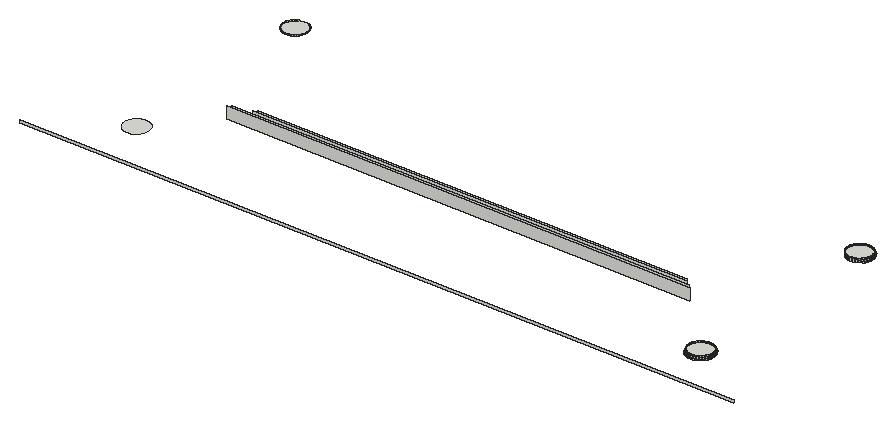
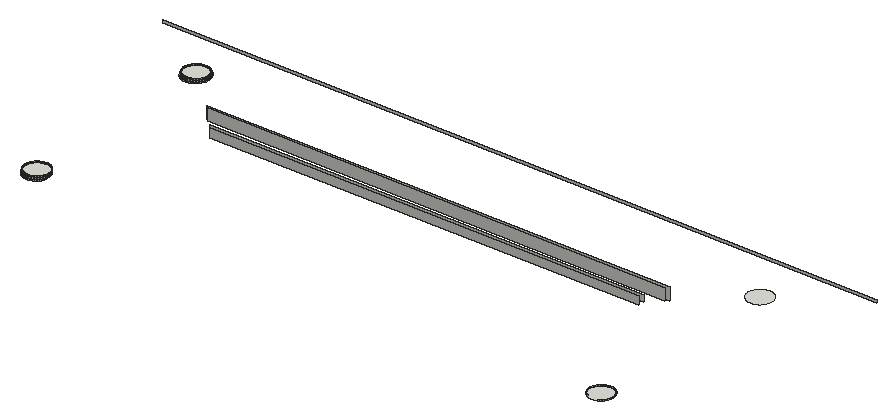
# SketchUp Ruby script. Lengths in inches.
U = 1.inch
M = Sketchup.active_model
def pt(a) = Geom::Point3d.new(a.map { |v| v * U })
def face(e, loops, mat)
  f = e.add_face(loops[0].map { |a| pt(a) })
  loops[1..].each { |l| e.add_face(l.map { |a| pt(a) }).erase! }
  f.material = f.back_material = mat if mat
  f
end
# faces: each face lists its corners as indices into pts; further lists are holes
def faces(e, pts, list, mat = nil) = list.each { |f| face(e, (f[0].is_a?(Array) ? f : [f]).map { |l| l.map { |i| pts[i] } }, mat) }
# xy, xz, yz: faces in a plane at the given z, y or x. An outline is a flat list of corners, or four numbers for a rectangle; further outlines are holes
def ring(l) = l.size == 4 ? [[l[0], l[1]], [l[2], l[1]], [l[2], l[3]], [l[0], l[3]]] : l.each_slice(2).to_a
def flat(e, list, mat, &to3) = list.each { |f| face(e, (f[0].is_a?(Array) ? f : [f]).map { |l| ring(l).map { |u, v| to3.(u, v) } }, mat) }
def xy(e, z, list, mat = nil) = flat(e, list, mat) { |x, y| [x, y, z] }
def xz(e, y, list, mat = nil) = flat(e, list, mat) { |x, z| [x, y, z] }
def yz(e, x, list, mat = nil) = flat(e, list, mat) { |y, z| [x, y, z] }
def lines(e, pts, list) = list.each { |a, b| e.add_line(pt(pts[a]), pt(pts[b])) }
# prism: a flat outline (further loops are holes) pulled along v
def prism(e, loops, v, mat = nil)
  f = face(e, loops, mat); d = Geom::Vector3d.new(v.map { |x| x * U })
  f.pushpull(f.normal.samedirection?(d) ? d.length : -d.length)
end
def box(e, o, s, mat = nil) = prism(e, [[o, [o[0] + s[0], o[1], o[2]], [o[0] + s[0], o[1] + s[1], o[2]], [o[0], o[1] + s[1], o[2]]]], [0, 0, s[2]], mat)
def at(x, y, z, deg = 0) = Geom::Transformation.translation(pt([x, y, z])) * Geom::Transformation.rotation(ORIGIN, Z_AXIS, deg.degrees)
def axes(o, x, y, z) = Geom::Transformation.new([*x, 0, *y, 0, *z, 0, *pt(o).to_a, 1])
def part(name) = M.definitions.add(name)
# library, detail: a bought-in or finely detailed component or shape, given as its bounding box
def library(name, o, s) = part(name).tap { |d| box(d.entities, o, s) }
def detail(e, o, s) = box(e.add_group.entities, o, s)
def put(e, d, t, mat = nil) = e.add_instance(d, t).tap { |i| i.material = mat if mat }
def group(e, t, mat = nil) = e.add_group.tap { |g| g.transformation = t; g.material = mat if mat }.entities
root = M.entities
xy(root,113.9,[[[112.03,5.8,111.8,5.81,111.57,5.84,111.35,5.9,111.13,5.98,110.92,6.08,110.73,6.2,110.55,6.35,110.38,6.51,110.24,6.69,110.11,6.875,110,7.08,109.92,7.29,109.85,7.52,109.82,7.74,109.8,7.97,109.81,8.2,109.84,8.43,109.9,8.65,109.98,8.87,110.08,9.08,110.2,9.27,110.35,9.45,110.51,9.62,110.69,9.76,110.875,9.89,111.08,10,111.29,10.08,111.52,10.15,111.74,10.18,111.97,10.2,112.2,10.19,112.43,10.16,112.65,10.1,112.87,10.02,113.08,9.92,113.27,9.8,113.45,9.65,113.62,9.49,113.76,9.31,113.89,9.125,114,8.92,114.08,8.71,114.15,8.48,114.18,8.26,114.2,8.03,114.19,7.8,114.16,7.57,114.1,7.35,114.02,7.13,113.92,6.92,113.8,6.73,113.65,6.55,113.49,6.38,113.31,6.24,113.125,6.11,112.92,6,112.71,5.92,112.48,5.85,112.26,5.82],[112.02,6,112.23,6.01,112.44,6.05,112.64,6.11,112.84,6.18,113.02,6.28,113.2,6.4,113.36,6.53,113.5,6.68,113.63,6.84,113.74,7.02,113.84,7.21,113.91,7.41,113.96,7.61,113.99,7.82,114,8.02,113.99,8.23,113.95,8.44,113.89,8.64,113.82,8.84,113.72,9.02,113.6,9.2,113.47,9.36,113.32,9.5,113.16,9.63,112.98,9.74,112.79,9.84,112.59,9.91,112.39,9.96,112.18,9.99,111.98,10,111.77,9.99,111.56,9.95,111.36,9.89,111.16,9.82,110.98,9.72,110.8,9.6,110.64,9.47,110.5,9.32,110.37,9.16,110.26,8.98,110.16,8.79,110.09,8.59,110.04,8.39,110.01,8.18,110,7.98,110.01,7.77,110.05,7.56,110.11,7.36,110.18,7.16,110.28,6.98,110.4,6.8,110.53,6.64,110.68,6.5,110.84,6.37,111.02,6.26,111.21,6.16,111.41,6.09,111.61,6.04,111.82,6.01]]])
xy(root,114.1875,[[16.69,6.57,16.48,6.59,16.28,6.62,16.08,6.67,15.88,6.75,15.7,6.85,15.53,6.96,15.36,7.09,15.22,7.24,15.09,7.4,14.98,7.58,14.88,7.77,14.81,7.96,14.76,8.16,14.72,8.37,14.71,8.58,14.73,8.78,14.76,8.99,14.82,9.19,14.89,9.38,14.99,9.57,15.1,9.74,15.23,9.9,15.38,10.05,15.54,10.18,15.72,10.29,15.91,10.39,16.1,10.46,16.3,10.51,16.51,10.54,16.72,10.55,16.92,10.54,17.13,10.51,17.33,10.45,17.52,10.38,17.71,10.28,17.88,10.17,18.04,10.04,18.19,9.89,18.32,9.72,18.43,9.55,18.53,9.36,18.6,9.17,18.65,8.97,18.68,8.76,18.69,8.55,18.68,8.34,18.65,8.14,18.59,7.9375,18.52,7.74,18.42,7.56,18.31,7.38,18.18,7.22,18.03,7.08,17.86,6.95,17.6875,6.83,17.5,6.74,17.31,6.67,17.11,6.61,16.9,6.58]])
xy(root,114.32,[[112.02,6,111.82,6.01,111.61,6.04,111.41,6.09,111.21,6.16,111.02,6.26,110.84,6.37,110.68,6.5,110.53,6.64,110.4,6.8,110.28,6.98,110.18,7.16,110.11,7.36,110.05,7.56,110.01,7.77,110,7.98,110.01,8.18,110.04,8.39,110.09,8.59,110.16,8.79,110.26,8.98,110.37,9.16,110.5,9.32,110.64,9.47,110.8,9.6,110.98,9.72,111.16,9.82,111.36,9.89,111.56,9.95,111.77,9.99,111.98,10,112.18,9.99,112.39,9.96,112.59,9.91,112.79,9.84,112.98,9.74,113.16,9.63,113.32,9.5,113.47,9.36,113.6,9.2,113.72,9.02,113.82,8.84,113.89,8.64,113.95,8.44,113.99,8.23,114,8.02,113.99,7.82,113.96,7.61,113.91,7.41,113.84,7.21,113.74,7.02,113.63,6.84,113.5,6.68,113.36,6.53,113.2,6.4,113.02,6.28,112.84,6.18,112.64,6.11,112.44,6.05,112.23,6.01],[112.02,39.41,111.82,39.42,111.61,39.45,111.41,39.5,111.21,39.58,111.02,39.67,110.84,39.78,110.68,39.91,110.53,40.06,110.4,40.22,110.28,40.39,110.18,40.58,110.11,40.77,110.05,40.97,110.01,41.18,110,41.39,110.01,41.6,110.04,41.81,110.09,42.01,110.16,42.21,110.26,42.39,110.37,42.57,110.5,42.73,110.64,42.88,110.8,43.02,110.98,43.13,111.16,43.23,111.36,43.31,111.56,43.37,111.77,43.4,111.98,43.41,112.18,43.41,112.39,43.375,112.59,43.32,112.79,43.25,112.98,43.16,113.16,43.05,113.32,42.92,113.47,42.77,113.6,42.61,113.72,42.44,113.82,42.25,113.89,42.06,113.95,41.85,113.99,41.65,114,41.4375,113.99,41.23,113.96,41.02,113.91,40.82,113.84,40.625,113.74,40.44,113.63,40.26,113.5,40.09,113.36,39.94,113.2,39.8125,113.02,39.69,112.84,39.6,112.64,39.52,112.44,39.46,112.23,39.43]])
xy(root,114.33,[[16.59,39.92,16.38,39.94,16.18,39.99,15.98,40.05,15.79,40.14,15.61,40.25,15.44,40.37,15.29,40.51,15.15,40.67,15.03,40.84,14.92,41.02,14.84,41.21,14.78,41.41,14.73,41.61,14.71,41.82,14.72,42.03,14.74,42.23,14.78,42.4375,14.85,42.64,14.93,42.83,15.04,43.01,15.16,43.17,15.3,43.33,15.46,43.47,15.63,43.59,15.81,43.69,16,43.78,16.2,43.84,16.4,43.88,16.61,43.9,16.82,43.9,17.03,43.88,17.23,43.83,17.43,43.77,17.62,43.68,17.8,43.58,17.97,43.45,18.12,43.3125,18.26,43.16,18.38,42.99,18.49,42.81,18.57,42.61,18.63,42.42,18.67,42.21,18.7,42,18.69,41.79,18.67,41.59,18.625,41.38,18.5625,41.1875,18.47,41,18.37,40.82,18.25,40.65,18.11,40.49,17.95,40.35,17.78,40.23,17.6,40.13,17.41,40.05,17.21,39.98,17,39.94,16.8,39.92]])
xz(root,0,[[4,114,124,114.47]])
xz(root,17.06,[[25.06,114.47,102.94,116.47]])
xz(root,17.53,[[25.53,114.47,102.47,116.47]])
xz(root,19.53,[[27.53,114.47,100.47,115.47]])
xz(root,20,[[28,114,100,115.47]])
xz(root,39.92,[[16.59,114.33,16.8,114.47]])
xz(root,43.41,[[111.98,113.9,112.18,114.32],[111.98,114.32,112.18,114.47]])
p = [[111.57,5.84,114],[111.35,5.9,114],[111.35,5.9,113.9],[111.57,5.84,113.9],[111.8,5.81,114],[111.8,5.81,113.9],
  [112.03,5.8,114],[112.03,5.8,113.9],[112.26,5.82,114],[112.26,5.82,113.9],[112.48,5.85,114],[112.48,5.85,113.9],
  [111.13,5.98,114],[111.13,5.98,113.9],[112.71,5.92,114],[112.71,5.92,113.9],[112.92,6,114],[112.92,6,113.9],
  [110.92,6.08,114],[110.92,6.08,113.9],[111.61,6.04,113.9],[111.41,6.09,113.9],[111.41,6.09,114.32],[111.61,6.04,114.32],
  [111.82,6.01,113.9],[111.82,6.01,114.32],[112.02,6,113.9],[112.02,6,114.32],[112.23,6.01,113.9],[112.23,6.01,114.32],
  [112.44,6.05,113.9],[112.44,6.05,114.32],[112.64,6.11,113.9],[112.64,6.11,114.32],[113.125,6.11,114],[113.125,6.11,113.9],
  [110.73,6.2,114],[110.73,6.2,113.9],[111.21,6.16,113.9],[111.21,6.16,114.32],[112.84,6.18,113.9],[112.84,6.18,114.32],
  [113.31,6.24,114],[113.31,6.24,113.9],[110.55,6.35,114],[110.55,6.35,113.9],[111.02,6.26,113.9],[111.02,6.26,114.32],
  [113.02,6.28,113.9],[113.02,6.28,114.32],[113.49,6.38,114],[113.49,6.38,113.9],[110.38,6.51,114],[110.38,6.51,113.9],
  [110.84,6.37,113.9],[110.84,6.37,114.32],[113.2,6.4,113.9],[113.2,6.4,114.32],[110.68,6.5,113.9],[110.68,6.5,114.32],
  [113.36,6.53,113.9],[113.36,6.53,114.32],[113.65,6.55,114],[113.65,6.55,113.9],[110.24,6.69,114],[110.24,6.69,113.9],
  [110.53,6.64,113.9],[110.53,6.64,114.32],[113.5,6.68,113.9],[113.5,6.68,114.32],[113.8,6.73,114],[113.8,6.73,113.9],
  [110.4,6.8,113.9],[110.4,6.8,114.32],[110.11,6.875,114],[110.11,6.875,113.9],[113.63,6.84,113.9],[113.63,6.84,114.32],
  [113.92,6.92,114],[113.92,6.92,113.9],[110.28,6.98,113.9],[110.28,6.98,114.32],[113.74,7.02,113.9],[113.74,7.02,114.32],
  [110,7.08,114],[110,7.08,113.9],[114.02,7.13,114],[114.02,7.13,113.9],[110.18,7.16,113.9],[110.18,7.16,114.32],
  [113.84,7.21,113.9],[113.84,7.21,114.32],[109.92,7.29,114],[109.92,7.29,113.9],[114.1,7.35,114],[114.1,7.35,113.9],
  [110.11,7.36,113.9],[110.11,7.36,114.32],[113.91,7.41,113.9],[113.91,7.41,114.32],[109.85,7.52,114],[109.85,7.52,113.9],
  [114.16,7.57,114],[114.16,7.57,113.9],[110.05,7.56,113.9],[110.05,7.56,114.32],[113.96,7.61,113.9],[113.96,7.61,114.32],
  [109.82,7.74,114],[109.82,7.74,113.9],[110.01,7.77,113.9],[110.01,7.77,114.32],[113.99,7.82,113.9],[113.99,7.82,114.32],
  [114.19,7.8,114],[114.19,7.8,113.9],[109.8,7.97,114],[109.8,7.97,113.9],[110,7.98,113.9],[110,7.98,114.32],
  [114,8.02,113.9],[114,8.02,114.32],[114.2,8.03,114],[114.2,8.03,113.9],[109.81,8.2,114],[109.81,8.2,113.9],
  [110.01,8.18,113.9],[110.01,8.18,114.32],[113.99,8.23,113.9],[113.99,8.23,114.32],[114.18,8.26,114],[114.18,8.26,113.9],
  [109.84,8.43,114],[109.84,8.43,113.9],[110.04,8.39,113.9],[110.04,8.39,114.32],[113.95,8.44,113.9],[113.95,8.44,114.32],
  [114.15,8.48,114],[114.15,8.48,113.9],[109.9,8.65,114],[109.9,8.65,113.9],[110.09,8.59,113.9],[110.09,8.59,114.32],
  [113.89,8.64,113.9],[113.89,8.64,114.32],[114.08,8.71,114],[114.08,8.71,113.9],[110.16,8.79,113.9],[110.16,8.79,114.32],
  [113.82,8.84,113.9],[113.82,8.84,114.32],[109.98,8.87,114],[109.98,8.87,113.9],[114,8.92,114],[114,8.92,113.9],
  [110.26,8.98,113.9],[110.26,8.98,114.32],[113.72,9.02,113.9],[113.72,9.02,114.32],[110.08,9.08,114],[110.08,9.08,113.9],
  [113.89,9.125,114],[113.89,9.125,113.9],[110.37,9.16,113.9],[110.37,9.16,114.32],[113.6,9.2,113.9],[113.6,9.2,114.32],
  [110.2,9.27,114],[110.2,9.27,113.9],[113.76,9.31,114],[113.76,9.31,113.9],[110.5,9.32,113.9],[110.5,9.32,114.32],
  [113.47,9.36,113.9],[113.47,9.36,114.32],[110.35,9.45,114],[110.35,9.45,113.9],[110.64,9.47,113.9],[110.64,9.47,114.32],
  [113.62,9.49,114],[113.62,9.49,113.9],[113.32,9.5,113.9],[113.32,9.5,114.32],[110.51,9.62,114],[110.51,9.62,113.9],
  [110.8,9.6,113.9],[110.8,9.6,114.32],[113.16,9.63,113.9],[113.16,9.63,114.32],[113.45,9.65,114],[113.45,9.65,113.9],
  [110.69,9.76,114],[110.69,9.76,113.9],[110.98,9.72,113.9],[110.98,9.72,114.32],[112.98,9.74,113.9],[112.98,9.74,114.32],
  [111.16,9.82,113.9],[111.16,9.82,114.32],[112.79,9.84,113.9],[112.79,9.84,114.32],[113.27,9.8,114],[113.27,9.8,113.9],
  [110.875,9.89,114],[110.875,9.89,113.9],[111.36,9.89,113.9],[111.36,9.89,114.32],[112.59,9.91,113.9],[112.59,9.91,114.32],
  [113.08,9.92,114],[113.08,9.92,113.9],[111.08,10,114],[111.08,10,113.9],[111.56,9.95,113.9],[111.56,9.95,114.32],
  [112.39,9.96,113.9],[112.39,9.96,114.32],[112.87,10.02,114],[112.87,10.02,113.9],[111.29,10.08,114],[111.29,10.08,113.9],
  [111.77,9.99,113.9],[111.77,9.99,114.32],[111.98,10,113.9],[111.98,10,114.32],[112.18,9.99,113.9],[112.18,9.99,114.32],
  [112.65,10.1,114],[112.65,10.1,113.9],[111.52,10.15,114],[111.52,10.15,113.9],[111.74,10.18,114],[111.74,10.18,113.9],
  [112.43,10.16,114],[112.43,10.16,113.9],[111.97,10.2,114],[111.97,10.2,113.9],[112.2,10.19,114],[112.2,10.19,113.9],
  [111.82,39.42,113.9],[111.61,39.45,113.9],[111.61,39.45,114.32],[111.82,39.42,114.32],[112.02,39.41,113.9],[112.02,39.41,114.32],
  [112.23,39.43,113.9],[112.23,39.43,114.32],[112.44,39.46,113.9],[112.44,39.46,114.32],[111.41,39.5,113.9],[111.21,39.58,113.9],
  [111.21,39.58,114.32],[111.41,39.5,114.32],[112.64,39.52,113.9],[112.64,39.52,114.32],[112.84,39.6,113.9],[112.84,39.6,114.32],
  [111.02,39.67,113.9],[111.02,39.67,114.32],[113.02,39.69,113.9],[113.02,39.69,114.32],[110.84,39.78,113.9],[110.84,39.78,114.32],
  [113.2,39.8125,113.9],[113.2,39.8125,114.32],[110.68,39.91,113.9],[110.68,39.91,114.32],[113.36,39.94,113.9],[113.36,39.94,114.32],
  [110.53,40.06,113.9],[110.53,40.06,114.32],[113.5,40.09,113.9],[113.5,40.09,114.32],[113.8,40.14,114],[113.65,39.96,114],
  [113.65,39.96,113.9],[113.8,40.14,113.9],[110.4,40.22,113.9],[110.4,40.22,114.32],[113.63,40.26,113.9],[113.63,40.26,114.32],
  [113.92,40.34,114],[113.92,40.34,113.9],[110.28,40.39,113.9],[110.28,40.39,114.32],[113.74,40.44,113.9],[113.74,40.44,114.32],
  [114.02,40.54,114],[114.02,40.54,113.9],[110.18,40.58,113.9],[110.18,40.58,114.32],[113.84,40.625,113.9],[113.84,40.625,114.32],
  [114.1,40.76,114],[114.1,40.76,113.9],[110.11,40.77,113.9],[110.11,40.77,114.32],[113.91,40.82,113.9],[113.91,40.82,114.32],
  [110.05,40.97,113.9],[110.05,40.97,114.32],[113.96,41.02,113.9],[113.96,41.02,114.32],[114.16,40.98,114],[114.16,40.98,113.9],
  [110.01,41.18,113.9],[110.01,41.18,114.32],[113.99,41.23,113.9],[113.99,41.23,114.32],[114.19,41.21,114],[114.19,41.21,113.9],
  [110,41.39,113.9],[110,41.39,114.32],[114,41.4375,113.9],[114,41.4375,114.32],[114.2,41.44,114],[114.2,41.44,113.9],
  [110.01,41.6,113.9],[110.01,41.6,114.32],[113.99,41.65,113.9],[113.99,41.65,114.32],[114.18,41.67,114],[114.18,41.67,113.9],
  [110.04,41.81,113.9],[110.04,41.81,114.32],[113.95,41.85,113.9],[113.95,41.85,114.32],[114.15,41.9,114],[114.15,41.9,113.9],
  [110.09,42.01,113.9],[110.09,42.01,114.32],[113.89,42.06,113.9],[113.89,42.06,114.32],[114.08,42.12,114],[114.08,42.12,113.9],
  [110.16,42.21,113.9],[110.16,42.21,114.32],[109.9,42.07,114],[109.98,42.28,114],[109.98,42.28,113.9],[109.9,42.07,113.9],
  [113.82,42.25,113.9],[113.82,42.25,114.32],[114,42.33,114],[114,42.33,113.9],[110.26,42.39,113.9],[110.26,42.39,114.32],
  [113.72,42.44,113.9],[113.72,42.44,114.32],[110.08,42.49,114],[110.08,42.49,113.9],[113.89,42.54,114],[113.89,42.54,113.9],
  [110.37,42.57,113.9],[110.37,42.57,114.32],[113.6,42.61,113.9],[113.6,42.61,114.32],[110.2,42.69,114],[110.2,42.69,113.9],
  [113.76,42.73,114],[113.76,42.73,113.9],[110.5,42.73,113.9],[110.5,42.73,114.32],[113.47,42.77,113.9],[113.47,42.77,114.32],
  [110.35,42.87,114],[110.35,42.87,113.9],[110.64,42.88,113.9],[110.64,42.88,114.32],[113.62,42.91,114],[113.62,42.91,113.9],
  [113.32,42.92,113.9],[113.32,42.92,114.32],[110.51,43.03,114],[110.51,43.03,113.9],[110.8,43.02,113.9],[110.8,43.02,114.32],
  [113.16,43.05,113.9],[113.16,43.05,114.32],[113.45,43.07,114],[113.45,43.07,113.9],[110.69,43.18,114],[110.69,43.18,113.9],
  [110.98,43.13,113.9],[110.98,43.13,114.32],[112.98,43.16,113.9],[112.98,43.16,114.32],[111.16,43.23,113.9],[111.16,43.23,114.32],
  [113.27,43.21,114],[113.27,43.21,113.9],[110.875,43.31,114],[110.875,43.31,113.9],[111.36,43.31,113.9],[111.36,43.31,114.32],
  [112.79,43.25,113.9],[112.79,43.25,114.32],[113.08,43.33,114],[113.08,43.33,113.9],[111.08,43.41,114],[111.08,43.41,113.9],
  [111.56,43.37,113.9],[111.56,43.37,114.32],[112.39,43.375,113.9],[112.59,43.32,113.9],[112.59,43.32,114.32],[112.39,43.375,114.32],
  [112.87,43.43,114],[112.87,43.43,113.9],[111.29,43.5,114],[111.29,43.5,113.9],[111.77,43.4,113.9],[111.77,43.4,114.32],
  [111.98,43.41,113.9],[111.98,43.41,114.32],[112.18,43.41,113.9],[112.18,43.41,114.32],[112.65,43.51,114],[112.65,43.51,113.9],
  [111.52,43.56,114],[111.52,43.56,113.9],[112.43,43.57,114],[112.43,43.57,113.9],[111.74,43.6,114],[111.74,43.6,113.9],
  [111.97,43.61,114],[111.97,43.61,113.9],[112.2,43.6,114],[112.2,43.6,113.9],[111.61,6.04,114.47],[111.41,6.09,114.47],
  [111.82,6.01,114.47],[112.02,6,114.47],[112.23,6.01,114.47],[112.44,6.05,114.47],[112.64,6.11,114.47],[111.21,6.16,114.47],
  [112.84,6.18,114.47],[111.02,6.26,114.47],[113.02,6.28,114.47],[110.84,6.37,114.47],[113.2,6.4,114.47],[110.68,6.5,114.47],
  [113.36,6.53,114.47],[110.53,6.64,114.47],[113.5,6.68,114.47],[110.4,6.8,114.47],[113.63,6.84,114.47],[110.28,6.98,114.47],
  [113.74,7.02,114.47],[110.18,7.16,114.47],[113.84,7.21,114.47],[110.11,7.36,114.47],[113.91,7.41,114.47],[110.05,7.56,114.47],
  [113.96,7.61,114.47],[110.01,7.77,114.47],[113.99,7.82,114.47],[110,7.98,114.47],[114,8.02,114.47],[110.01,8.18,114.47],
  [113.99,8.23,114.47],[110.04,8.39,114.47],[113.95,8.44,114.47],[110.09,8.59,114.47],[113.89,8.64,114.47],[110.16,8.79,114.47],
  [113.82,8.84,114.47],[110.26,8.98,114.47],[113.72,9.02,114.47],[110.37,9.16,114.47],[113.6,9.2,114.47],[110.5,9.32,114.47],
  [113.47,9.36,114.47],[110.64,9.47,114.47],[113.32,9.5,114.47],[110.8,9.6,114.47],[113.16,9.63,114.47],[110.98,9.72,114.47],
  [112.98,9.74,114.47],[111.16,9.82,114.47],[112.79,9.84,114.47],[111.36,9.89,114.47],[112.59,9.91,114.47],[111.56,9.95,114.47],
  [112.39,9.96,114.47],[111.77,9.99,114.47],[111.98,10,114.47],[112.18,9.99,114.47],[111.82,39.42,114.47],[111.61,39.45,114.47],
  [112.02,39.41,114.47],[112.23,39.43,114.47],[112.44,39.46,114.47],[111.41,39.5,114.47],[111.21,39.58,114.47],[112.64,39.52,114.47],
  [112.84,39.6,114.47],[111.02,39.67,114.47],[113.02,39.69,114.47],[110.84,39.78,114.47],[113.2,39.8125,114.47],[110.68,39.91,114.47],
  [113.36,39.94,114.47],[16.38,39.94,114.47],[16.38,39.94,114.33],[16.18,39.99,114.33],[16.18,39.99,114.47],[16.59,39.92,114.47],
  [16.59,39.92,114.33],[17,39.94,114.47],[17,39.94,114.33],[16.8,39.92,114.33],[16.8,39.92,114.47],[17.21,39.98,114.47],
  [17.21,39.98,114.33],[110.53,40.06,114.47],[113.5,40.09,114.47],[15.98,40.05,114.33],[15.98,40.05,114.47],[17.41,40.05,114.47],
  [17.41,40.05,114.33],[17.6,40.13,114.47],[17.6,40.13,114.33],[15.79,40.14,114.47],[15.79,40.14,114.33],[15.61,40.25,114.33],
  [15.61,40.25,114.47],[17.78,40.23,114.47],[17.78,40.23,114.33],[110.4,40.22,114.47],[113.63,40.26,114.47],[15.44,40.37,114.33],
  [15.44,40.37,114.47],[17.95,40.35,114.47],[17.95,40.35,114.33],[110.28,40.39,114.47],[113.74,40.44,114.47],[15.29,40.51,114.33],
  [15.29,40.51,114.47],[18.11,40.49,114.47],[18.11,40.49,114.33],[110.18,40.58,114.47],[113.84,40.625,114.47],[15.15,40.67,114.33],
  [15.15,40.67,114.47],[18.25,40.65,114.47],[18.25,40.65,114.33],[18.37,40.82,114.47],[18.37,40.82,114.33],[110.11,40.77,114.47],
  [113.91,40.82,114.47],[15.03,40.84,114.33],[15.03,40.84,114.47],[14.92,41.02,114.33],[14.92,41.02,114.47],[18.47,41,114.47],
  [18.47,41,114.33],[110.05,40.97,114.47],[113.96,41.02,114.47],[14.84,41.21,114.33],[14.84,41.21,114.47],[18.5625,41.1875,114.47],
  [18.5625,41.1875,114.33],[110.01,41.18,114.47],[113.99,41.23,114.47],[14.78,41.41,114.33],[14.78,41.41,114.47],[18.625,41.38,114.47],
  [18.625,41.38,114.33],[110,41.39,114.47],[114,41.4375,114.47],[14.73,41.61,114.33],[14.73,41.61,114.47],[18.67,41.59,114.47],
  [18.67,41.59,114.33],[110.01,41.6,114.47],[113.99,41.65,114.47],[14.71,41.82,114.33],[14.71,41.82,114.47],[18.69,41.79,114.47],
  [18.69,41.79,114.33],[110.04,41.81,114.47],[113.95,41.85,114.47],[14.72,42.03,114.33],[14.72,42.03,114.47],[18.7,42,114.47],
  [18.7,42,114.33],[110.09,42.01,114.47],[113.89,42.06,114.47],[14.74,42.23,114.33],[14.74,42.23,114.47],[18.67,42.21,114.47],
  [18.67,42.21,114.33],[110.16,42.21,114.47],[113.82,42.25,114.47],[14.78,42.4375,114.33],[14.78,42.4375,114.47],[18.63,42.42,114.47],
  [18.63,42.42,114.33],[110.26,42.39,114.47],[113.72,42.44,114.47],[14.85,42.64,114.33],[14.85,42.64,114.47],[18.57,42.61,114.47],
  [18.57,42.61,114.33],[110.37,42.57,114.47],[113.6,42.61,114.47],[14.93,42.83,114.33],[14.93,42.83,114.47],[18.49,42.81,114.47],
  [18.49,42.81,114.33],[110.5,42.73,114.47],[113.47,42.77,114.47],[110.64,42.88,114.47],[15.04,43.01,114.33],[15.04,43.01,114.47],
  [18.38,42.99,114.47],[18.38,42.99,114.33],[113.32,42.92,114.47],[110.8,43.02,114.47],[113.16,43.05,114.47],[15.16,43.17,114.33],
  [15.16,43.17,114.47],[18.26,43.16,114.47],[18.26,43.16,114.33],[110.98,43.13,114.47],[112.98,43.16,114.47],[111.16,43.23,114.47],
  [15.3,43.33,114.33],[15.3,43.33,114.47],[18.12,43.3125,114.47],[18.12,43.3125,114.33],[111.36,43.31,114.47],[112.79,43.25,114.47],
  [15.46,43.47,114.33],[15.46,43.47,114.47],[17.97,43.45,114.47],[17.97,43.45,114.33],[111.56,43.37,114.47],[112.39,43.375,114.47],
  [112.59,43.32,114.47],[111.77,43.4,114.47],[111.98,43.41,114.47],[112.18,43.41,114.47],[15.63,43.59,114.33],[15.63,43.59,114.47],
  [17.8,43.58,114.47],[17.8,43.58,114.33],[15.81,43.69,114.33],[15.81,43.69,114.47],[17.62,43.68,114.47],[17.62,43.68,114.33]]
faces(root,p,[[0,1,2,3],[4,0,3,5],[6,4,5,7],[8,6,7,9],[10,8,9,11],[1,12,13,2],[14,10,11,15],[16,14,15,17],
  [12,18,19,13],[20,21,22,23],[24,20,23,25],[26,24,25,27],[28,26,27,29],[30,28,29,31],[32,30,31,33],[34,16,17,35],
  [18,36,37,19],[21,38,39,22],[40,32,33,41],[42,34,35,43],[36,44,45,37],[38,46,47,39],[48,40,41,49],[50,42,43,51],
  [44,52,53,45],[46,54,55,47],[56,48,49,57],[54,58,59,55],[60,56,57,61],[62,50,51,63],[52,64,65,53],[58,66,67,59],
  [68,60,61,69],[70,62,63,71],[66,72,73,67],[64,74,75,65],[76,68,69,77],[78,70,71,79],[72,80,81,73],[82,76,77,83],
  [74,84,85,75],[86,78,79,87],[80,88,89,81],[90,82,83,91],[84,92,93,85],[94,86,87,95],[88,96,97,89],[98,90,91,99],
  [92,100,101,93],[102,94,95,103],[96,104,105,97],[106,98,99,107],[100,108,109,101],[104,110,111,105],[112,106,107,113],[114,102,103,115],
  [108,116,117,109],[110,118,119,111],[120,112,113,121],[122,114,115,123],[116,124,125,117],[118,126,127,119],[128,120,121,129],[130,122,123,131],
  [124,132,133,125],[126,134,135,127],[136,128,129,137],[138,130,131,139],[132,140,141,133],[134,142,143,135],[144,136,137,145],[146,138,139,147],
  [142,148,149,143],[150,144,145,151],[140,152,153,141],[154,146,147,155],[148,156,157,149],[158,150,151,159],[152,160,161,153],[162,154,155,163],
  [156,164,165,157],[166,158,159,167],[160,168,169,161],[170,162,163,171],[164,172,173,165],[174,166,167,175],[168,176,177,169],[172,178,179,173],
  [180,170,171,181],[182,174,175,183],[176,184,185,177],[178,186,187,179],[188,182,183,189],[190,180,181,191],[184,192,193,185],[186,194,195,187],
  [196,188,189,197],[194,198,199,195],[200,196,197,201],[202,190,191,203],[192,204,205,193],[198,206,207,199],[208,200,201,209],[210,202,203,211],
  [204,212,213,205],[206,214,215,207],[216,208,209,217],[218,210,211,219],[212,220,221,213],[214,222,223,215],[222,224,225,223],[224,226,227,225],
  [226,216,217,227],[228,218,219,229],[220,230,231,221],[230,232,233,231],[234,228,229,235],[232,236,237,233],[236,238,239,237],[238,234,235,239],
  [240,241,242,243],[244,240,243,245],[246,244,245,247],[248,246,247,249],[250,251,252,253],[241,250,253,242],[254,248,249,255],[256,254,255,257],
  [251,258,259,252],[260,256,257,261],[258,262,263,259],[264,260,261,265],[262,266,267,263],[268,264,265,269],[266,270,271,267],[272,268,269,273],
  [274,275,276,277],[270,278,279,271],[280,272,273,281],[282,274,277,283],[278,284,285,279],[286,280,281,287],[288,282,283,289],[284,290,291,285],
  [292,286,287,293],[294,288,289,295],[290,296,297,291],[298,292,293,299],[296,300,301,297],[302,298,299,303],[304,294,295,305],[300,306,307,301],
  [308,302,303,309],[310,304,305,311],[306,312,313,307],[314,308,309,315],[316,310,311,317],[312,318,319,313],[320,314,315,321],[322,316,317,323],
  [318,324,325,319],[326,320,321,327],[328,322,323,329],[324,330,331,325],[332,326,327,333],[334,328,329,335],[330,336,337,331],[338,339,340,341],
  [342,332,333,343],[344,334,335,345],[336,346,347,337],[348,342,343,349],[339,350,351,340],[352,344,345,353],[346,354,355,347],[356,348,349,357],
  [350,358,359,351],[360,352,353,361],[354,362,363,355],[364,356,357,365],[358,366,367,359],[362,368,369,363],[370,360,361,371],[372,364,365,373],
  [366,374,375,367],[368,376,377,369],[378,372,373,379],[380,370,371,381],[374,382,383,375],[376,384,385,377],[386,378,379,387],[384,388,389,385],
  [390,380,381,391],[382,392,393,383],[388,394,395,389],[396,386,387,397],[398,390,391,399],[392,400,401,393],[394,402,403,395],[404,405,406,407],
  [405,396,397,406],[408,398,399,409],[400,410,411,401],[402,412,413,403],[412,414,415,413],[416,404,407,417],[418,408,409,419],[410,420,421,411],
  [422,418,419,423],[420,424,425,421],[424,426,427,425],[426,428,429,427],[428,422,423,429],[430,23,22,431],[432,25,23,430],[433,27,25,432],
  [434,29,27,433],[435,31,29,434],[436,33,31,435],[431,22,39,437],[438,41,33,436],[437,39,47,439],[440,49,41,438],[439,47,55,441],
  [442,57,49,440],[441,55,59,443],[444,61,57,442],[443,59,67,445],[446,69,61,444],[445,67,73,447],[448,77,69,446],[447,73,81,449],
  [450,83,77,448],[449,81,89,451],[452,91,83,450],[451,89,97,453],[454,99,91,452],[453,97,105,455],[456,107,99,454],[455,105,111,457],
  [458,113,107,456],[457,111,119,459],[460,121,113,458],[459,119,127,461],[462,129,121,460],[461,127,135,463],[464,137,129,462],[463,135,143,465],
  [466,145,137,464],[465,143,149,467],[468,151,145,466],[467,149,157,469],[470,159,151,468],[469,157,165,471],[472,167,159,470],[471,165,173,473],
  [474,175,167,472],[473,173,179,475],[476,183,175,474],[475,179,187,477],[478,189,183,476],[477,187,195,479],[480,197,189,478],[479,195,199,481],
  [482,201,197,480],[481,199,207,483],[484,209,201,482],[483,207,215,485],[486,217,209,484],[485,215,223,487],[487,223,225,488],[488,225,227,489],
  [489,227,217,486],[490,243,242,491],[492,245,243,490],[493,247,245,492],[494,249,247,493],[495,253,252,496],[491,242,253,495],[497,255,249,494],
  [498,257,255,497],[496,252,259,499],[500,261,257,498],[499,259,263,501],[502,265,261,500],[501,263,267,503],[504,269,265,502],[505,506,507,508],
  [509,510,506,505],[511,512,513,514],[515,516,512,511],[503,267,271,517],[518,273,269,504],[508,507,519,520],[521,522,516,515],[523,524,522,521],
  [525,526,527,528],[520,519,526,525],[529,530,524,523],[517,271,279,531],[532,281,273,518],[528,527,533,534],[535,536,530,529],[531,279,285,537],
  [538,287,281,532],[534,533,539,540],[541,542,536,535],[537,285,291,543],[544,293,287,538],[540,539,545,546],[547,548,542,541],[549,550,548,547],
  [543,291,297,551],[552,299,293,544],[546,545,553,554],[554,553,555,556],[557,558,550,549],[551,297,301,559],[560,303,299,552],[556,555,561,562],
  [563,564,558,557],[559,301,307,565],[566,309,303,560],[562,561,567,568],[569,570,564,563],[565,307,313,571],[572,315,309,566],[568,567,573,574],
  [575,576,570,569],[571,313,319,577],[578,321,315,572],[574,573,579,580],[581,582,576,575],[577,319,325,583],[584,327,321,578],[580,579,585,586],
  [587,588,582,581],[583,325,331,589],[590,333,327,584],[586,585,591,592],[593,594,588,587],[589,331,337,595],[596,343,333,590],[592,591,597,598],
  [599,600,594,593],[595,337,347,601],[602,349,343,596],[598,597,603,604],[605,606,600,599],[601,347,355,607],[608,357,349,602],[604,603,609,610],
  [611,612,606,605],[607,355,363,613],[614,365,357,608],[613,363,369,615],[610,609,616,617],[618,619,612,611],[620,373,365,614],[615,369,377,621],
  [622,379,373,620],[617,616,623,624],[625,626,619,618],[621,377,385,627],[628,387,379,622],[627,385,389,629],[624,623,630,631],[632,633,626,625],
  [629,389,395,634],[635,397,387,628],[631,630,636,637],[638,639,633,632],[634,395,403,640],[641,407,406,642],[642,406,397,635],[640,403,413,643],
  [643,413,415,644],[645,417,407,641],[637,636,646,647],[648,649,639,638],[647,646,650,651],[652,653,649,648]])
